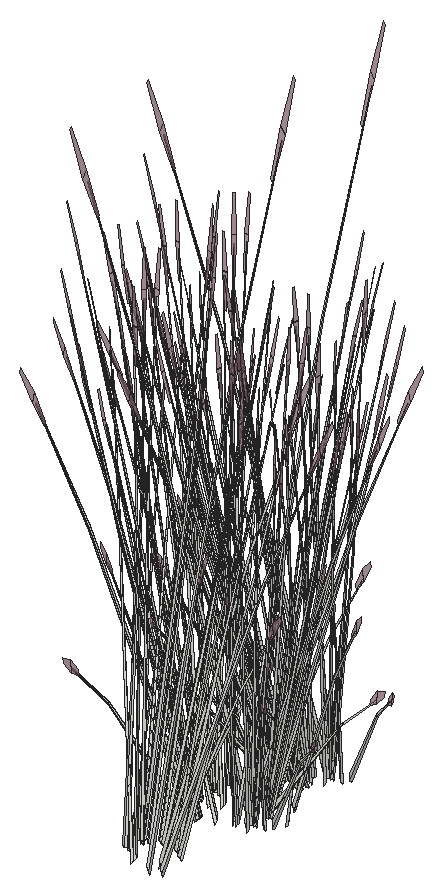
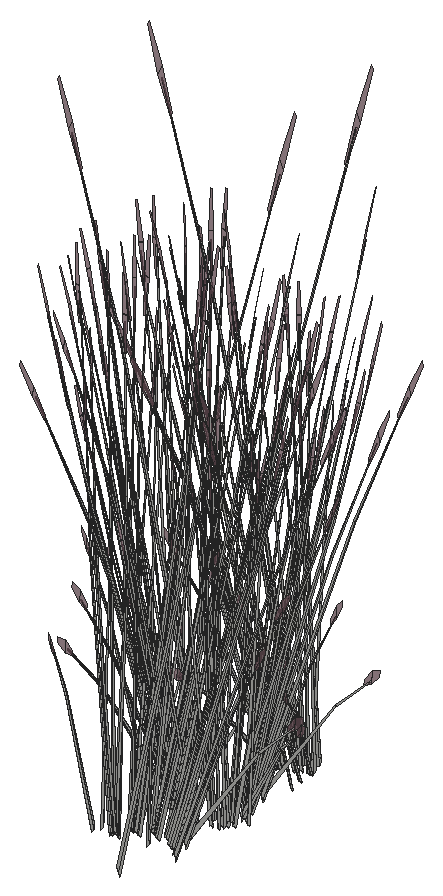
# SketchUp Ruby script. Lengths in inches.
U = 1.inch
M = Sketchup.active_model
def pt(a) = Geom::Point3d.new(a.map { |v| v * U })
def face(e, loops, mat)
  f = e.add_face(loops[0].map { |a| pt(a) })
  loops[1..].each { |l| e.add_face(l.map { |a| pt(a) }).erase! }
  f.material = f.back_material = mat if mat
  f
end
# faces: each face lists its corners as indices into pts; further lists are holes
def faces(e, pts, list, mat = nil) = list.each { |f| face(e, (f[0].is_a?(Array) ? f : [f]).map { |l| l.map { |i| pts[i] } }, mat) }
# xy, xz, yz: faces in a plane at the given z, y or x. An outline is a flat list of corners, or four numbers for a rectangle; further outlines are holes
def ring(l) = l.size == 4 ? [[l[0], l[1]], [l[2], l[1]], [l[2], l[3]], [l[0], l[3]]] : l.each_slice(2).to_a
def flat(e, list, mat, &to3) = list.each { |f| face(e, (f[0].is_a?(Array) ? f : [f]).map { |l| ring(l).map { |u, v| to3.(u, v) } }, mat) }
def xy(e, z, list, mat = nil) = flat(e, list, mat) { |x, y| [x, y, z] }
def xz(e, y, list, mat = nil) = flat(e, list, mat) { |x, z| [x, y, z] }
def yz(e, x, list, mat = nil) = flat(e, list, mat) { |y, z| [x, y, z] }
def lines(e, pts, list) = list.each { |a, b| e.add_line(pt(pts[a]), pt(pts[b])) }
# prism: a flat outline (further loops are holes) pulled along v
def prism(e, loops, v, mat = nil)
  f = face(e, loops, mat); d = Geom::Vector3d.new(v.map { |x| x * U })
  f.pushpull(f.normal.samedirection?(d) ? d.length : -d.length)
end
def box(e, o, s, mat = nil) = prism(e, [[o, [o[0] + s[0], o[1], o[2]], [o[0] + s[0], o[1] + s[1], o[2]], [o[0], o[1] + s[1], o[2]]]], [0, 0, s[2]], mat)
def at(x, y, z, deg = 0) = Geom::Transformation.translation(pt([x, y, z])) * Geom::Transformation.rotation(ORIGIN, Z_AXIS, deg.degrees)
def axes(o, x, y, z) = Geom::Transformation.new([*x, 0, *y, 0, *z, 0, *pt(o).to_a, 1])
def part(name) = M.definitions.add(name)
# library, detail: a bought-in or finely detailed component or shape, given as its bounding box
def library(name, o, s) = part(name).tap { |d| box(d.entities, o, s) }
def detail(e, o, s) = box(e.add_group.entities, o, s)
def put(e, d, t, mat = nil) = e.add_instance(d, t).tap { |i| i.material = mat if mat }
def group(e, t, mat = nil) = e.add_group.tap { |g| g.transformation = t; g.material = mat if mat }.entities
root = M.entities
M.materials.add("LightPink_Translucent").color = [144, 107, 117]
M.materials["LightPink_Translucent"].alpha = 0.75
c1 = part("blade")
p = [[2.15,0.21,22],[0,0.17,0],[0.09,0.45,0],[2.18,0.31,22],[2.29,0.31,22],[0.38,0.45,0],
  [2.48,0.24,33],[2.49,0.24,33],[2.48,0.22,33]]
faces(c1.entities,p,[[0,1,2,3],[4,5,2,3],[6,3,4,7],[8,0,3,6]])
c2 = part("seeds")
p = [[0.3,-0.1,1.38],[-0.01,-0.03,1.59],[-0.01,-0.03,0.03],[0.14,-0.07,-0.07],[0.29,-0.03,3],[0.15,0.01,3.11]]
faces(c2.entities,p,[[0,1,2,3],[1,0,4,5]],"LightPink_Translucent")
c3 = part("blade with seeds")
put(c3.entities,c1,at(0,0,0))
put(c3.entities,c2,axes([2.4,0.25,30.99],[1.5799,-0.05474,1.17369],[-0.12525,1.92788,0.29478],[-0.07173,-0.02425,1.56792]))
put(root,c3,axes([428.51,484.51,154],[0.18625,-0.29962,0.05432],[0.26523,0.17444,0.42765],[-0.08575,-0.09606,0.65209]))
put(root,c3,axes([427.57,485.1,153.27],[0.15222,0.08126,1.44779],[-0.31502,0.34091,0.11706],[-0.19634,-0.15379,0.61892]))
put(root,c3,axes([429.86,479.9,153.27],[-0.15222,-0.08126,1.44779],[0.31502,-0.34091,0.11706],[0.19634,0.15379,0.61892]))
put(root,c3,axes([429.88,478.83,153.78],[-0.35411,-0.24507,1.16821],[0.37391,-0.38156,0.50405],[0.11425,0.22994,1.12919]))
put(root,c3,axes([427.33,479.87,154.25],[0.37908,0.26007,-0.10273],[-0.21839,0.37663,-0.57019],[-0.1071,0.13092,0.8664]))
put(root,c3,axes([428.31,484.86,153.95],[-0.40438,0.11212,-0.43168],[-0.07074,-0.4246,-0.33437],[-0.10862,-0.12168,0.82598]))
put(root,c3,axes([430.35,484.95,154],[0.29182,0.32181,0.40553],[-0.3099,0.27755,0.33437],[0.05383,-0.15098,0.83914]))
put(root,c3,axes([429.61,481.22,154.25],[0.2442,-0.40372,-0.10273],[0.35364,0.23259,-0.57019],[0.12293,0.11406,0.8664]))
put(root,c3,axes([428.59,484.48,154.59],[-0.2735,0.45217,-0.11506],[-0.39608,-0.2605,-0.63862],[-0.13768,-0.12775,0.97037]))
put(root,c3,axes([430.46,484.98,154],[0.33677,0.02198,0.05432],[-0.00923,0.33185,0.42765],[0.03524,-0.12712,0.65209]))
put(root,c3,axes([427.84,479.75,153.27],[0.10236,-0.14492,1.44779],[0.25844,0.39118,0.11706],[-0.17726,0.17814,0.61892]))
put(root,c3,axes([427.52,480.18,153.95],[0.10528,0.43067,-0.43168],[-0.39868,0.07534,-0.33437],[-0.11425,0.11568,0.82598]))
put(root,c3,axes([430.7,485.87,154.21],[0.21406,-0.37215,-0.60019],[0.37511,0.26448,0.07243],[0.12781,-0.13483,0.84903]))
put(root,c3,axes([430.6875,485.7,153.95],[-0.10528,-0.43067,-0.43168],[0.39868,-0.07534,-0.33437],[0.11425,-0.11568,0.82598]))
put(root,c3,axes([429.29,481.55,153.98],[0.00121,-0.0571,1.49853],[0.35119,-0.25193,-0.1416],[0.12199,0.08992,0.26519]))
put(root,c3,axes([427.75,480.9,154],[-0.33677,-0.02198,0.05432],[0.00923,-0.33185,0.42765],[-0.03524,0.12712,0.65209]))
put(root,c3,axes([427.85,480.93,154],[-0.29182,-0.32181,0.40553],[0.3099,-0.27755,0.33437],[-0.05383,0.15098,0.83914]))
put(root,c3,axes([429.9,481.02,153.95],[0.40438,-0.11212,-0.43168],[0.07074,0.4246,-0.33437],[0.10862,0.12168,0.82598]))
put(root,c3,axes([427.54,484.35,153.98],[-0.08817,-0.00333,1.47793],[-0.28072,0.33293,-0.23373],[-0.14978,-0.06803,0.11853]))
put(root,c3,axes([430.875,486.01,154.25],[-0.37908,-0.26007,-0.10273],[0.21839,-0.37663,-0.57019],[0.1071,-0.13092,0.8664]))
put(root,c3,axes([429.31,487.43,152.81],[0.35414,0.19019,1.27785],[-0.34693,0.40974,0.50532],[-0.1554,-0.24285,1.07126]))
put(root,c3,axes([429.7,481.36,154],[-0.18625,0.29962,0.05432],[-0.26523,-0.17444,0.42765],[0.08575,0.09606,0.65209]))
put(root,c3,axes([431.81,485.89,153.98],[-0.05353,-0.00358,1.49853],[-0.22227,-0.38383,-0.1416],[0.08926,-0.1262,0.26519]))
put(root,c3,axes([429.78,481.28,154],[-0.4076,0.10824,0.40553],[-0.07074,-0.4246,0.33437],[0.09586,0.12514,0.83914]))
put(root,c3,axes([427.77,480.11,153.27],[0.0763,-0.16212,1.44779],[0.3201,0.3355,0.11706],[-0.1444,0.2091,0.61892]))
put(root,c3,axes([430.98,485.74,153.82],[0.35672,-0.06741,-0.29918],[0.09419,0.38534,0.38624],[0.10222,-0.1035,0.73904]))
put(root,c3,axes([427.63,485.1,154],[0.02064,-0.35866,0.05432],[0.3116,0.00983,0.42765],[-0.11936,-0.03753,0.65209]))
put(root,c3,axes([428.66,481.41,154],[-0.30197,0.1603,0.05432],[-0.1478,-0.29231,0.42765],[0.02916,0.12885,0.65209]))
put(root,c3,axes([427.85,481.02,153.82],[-0.27728,0.24833,-0.29918],[-0.26248,-0.28355,0.38624],[-0.03994,0.14407,0.73904]))
put(root,c3,axes([426.9,480.95,153.98],[-0.01019,0.09334,1.47793],[0.28908,0.3247,-0.23373],[-0.07568,0.15355,0.11853]))
put(root,c3,axes([427.82,480.74,154.56],[0.45039,0.02337,-0.11403],[-0.01231,0.44247,-0.63292],[-0.03129,0.17041,0.9617]))
put(root,c3,axes([427.51,485.21,153.82],[-0.23317,-0.29531,-0.29918],[0.26625,-0.27955,0.38624],[-0.13527,-0.04253,0.73904]))
put(root,c3,axes([428.66,481.23,154.25],[0.40102,-0.2196,-0.10273],[0.19707,0.38974,-0.57019],[0.05291,0.16424,0.8664]))
put(root,c3,axes([428.13,480.91,154.23],[0.29336,0.31691,-0.47917],[-0.3099,0.27755,-0.37115],[-0.04464,0.16102,0.91684]))
put(root,c3,axes([427.76,485.41,154.21],[-0.40965,-0.01136,-0.60019],[0.02751,-0.47821,0.07243],[-0.17355,-0.05047,0.84903]))
put(root,c3,axes([429,481.21,153.95],[0.40284,0.11824,-0.43168],[-0.13808,0.40538,-0.33437],[0.03694,0.16321,0.82598]))
put(root,c3,axes([429.23,480.375,153.27],[-0.09368,-0.15143,1.44779],[0.43286,-0.12749,0.11706],[0.09783,0.23774,0.61892]))
put(root,c3,axes([431.01,485.91,154],[0.28133,0.19836,0.05432],[-0.16379,0.28248,0.42765],[0.0902,-0.09132,0.65209]))
put(root,c3,axes([428.82,481.46,153.82],[-0.12355,0.36271,-0.29918],[-0.36044,-0.10579,0.38624],[0.03305,0.14603,0.73904]))
put(root,c3,axes([430.93,485.83,154],[0.10163,0.43409,0.40553],[-0.39868,0.07534,0.33437],[0.1175,-0.10209,0.83914]))
put(root,c3,axes([432.01,486.35,153.98],[0.05687,-0.07184,1.47793],[-0.07279,-0.44069,-0.23373],[0.14268,-0.08356,0.11853]))
put(root,c3,axes([428.04,480.76,154.51],[-0.01066,0.43628,-0.66621],[-0.44902,-0.0293,0.0804],[-0.04739,0.18483,0.94242]))
put(root,c3,axes([426.87,481.91,153.98],[0.04649,-0.02848,1.49853],[0.38427,0.18941,-0.1416],[-0.00903,0.15771,0.26519]))
put(root,c3,axes([427.2,484.63,153.98],[0.03038,0.04707,1.49853],[-0.14646,0.42312,-0.1416],[-0.14833,0.00306,0.26519]))
put(root,c3,axes([428.46,480.45,153.27],[-0.01003,-0.18103,1.44779],[0.43473,0.12009,0.11706],[-0.02689,0.25798,0.61892]))
put(root,c3,axes([427.625,485.51,153.95],[-0.29757,0.31243,-0.43168],[-0.2606,-0.33005,-0.33437],[-0.15119,-0.04754,0.82598]))
put(root,c3,axes([428.5625,482.1,153.98],[0.05195,0.07595,1.47793],[0.41921,0.02984,-0.23373],[0.04216,0.1675,0.11853]))
put(root,c3,axes([427.78,485.18,154.25],[-0.02194,0.47967,-0.10273],[-0.41546,-0.01311,-0.57019],[-0.16001,-0.03332,0.8664]))
put(root,c3,axes([430.89,487.02,154.25],[-0.20619,-0.42709,-0.10273],[0.36595,-0.20988,-0.57019],[0.15422,-0.05635,0.8664]))
put(root,c3,axes([430.87,486.65,153.95],[0.11102,-0.42903,-0.43168],[0.38064,0.14706,-0.33437],[0.15325,-0.03934,0.82598]))
put(root,c3,axes([427.25,485.84,153.27],[0.16998,-0.01068,1.44779],[-0.11276,0.46299,0.11706],[-0.24224,-0.02864,0.61892]))
put(root,c3,axes([430.8,486.81,154.21],[0.3601,-0.20831,-0.60019],[0.20068,0.4288,0.07243],[0.17399,-0.04871,0.84903]))
put(root,c3,axes([427.89,481.375,152.84],[0.009,-0.24349,1.30391],[0.40497,0.12861,0.18019],[-0.03509,0.2595,0.61571]))
put(root,c3,axes([427.18,486.19,154],[0.11578,-0.43006,0.40553],[0.38064,0.14706,0.33437],[-0.14969,0.02584,0.83914]))
put(root,c3,axes([427.15,486.08,154],[-0.15051,-0.3216,0.05432],[0.27447,-0.15741,0.42765],[-0.12099,0.03106,0.65209]))
put(root,c3,axes([431.1,486.85,153.82],[0.34057,0.13158,-0.29918],[-0.09933,0.38387,0.38624],[0.13712,-0.0352,0.73904]))
put(root,c3,axes([427.1,486.24,153.82],[-0.34057,-0.13158,-0.29918],[0.09933,-0.38387,0.38624],[-0.13712,0.0352,0.73904]))
put(root,c3,axes([428.2,490.79,153.27],[0.09368,0.15143,1.44779],[-0.43286,0.12749,0.11706],[-0.09783,-0.23774,0.61892]))
put(root,c3,axes([430.18,486.375,153.27],[-0.16998,0.01068,1.44779],[0.11276,-0.46299,0.11706],[0.24224,0.02864,0.61892]))
put(root,c3,axes([428.91,489.79,153.98],[-0.06268,-0.06613,1.47793],[-0.4183,0.04193,-0.23373],[-0.06676,-0.15817,0.11853]))
put(root,c3,axes([431.05,487.01,154],[0.15051,0.3216,0.05432],[-0.27447,0.15741,0.42765],[0.12099,-0.03106,0.65209]))
put(root,c3,axes([429.35,490.9,154.21],[-0.19559,-0.38351,-0.60019],[0.40262,-0.21373,0.07243],[-0.04574,-0.1853,0.84903]))
put(root,c3,axes([431.03,486.9,154],[-0.11578,0.43006,0.40553],[-0.38064,-0.14706,0.33437],[0.14969,-0.02584,0.83914]))
put(root,c3,axes([430.17,491.28,154.21],[0.01066,-0.43628,-0.60019],[0.44902,0.0293,0.07243],[0.04739,-0.18483,0.84903]))
put(root,c3,axes([428.14,486.17,152.82],[0.11649,-0.06823,1.49584],[0.04017,0.47639,0.11706],[-0.25231,0.06321,0.53462]))
put(root,c3,axes([430.79,490.6,153.98],[-0.00396,-0.09387,1.47793],[-0.33411,-0.2713,-0.23373],[0.05166,-0.16446,0.11853]))
put(root,c3,axes([429.39,490.58,153.82],[0.12355,-0.36271,-0.29918],[0.36044,0.10579,0.38624],[-0.03305,-0.14603,0.73904]))
put(root,c3,axes([429.66,491.06,153.27],[-0.0763,0.16212,1.44779],[-0.3201,-0.3355,0.11706],[0.1444,-0.2091,0.61892]))
put(root,c3,axes([430.7,490.26,153.98],[-0.04162,0.03603,1.49853],[-0.40776,-0.12155,-0.1416],[-0.01476,-0.15722,0.26519]))
put(root,c3,axes([429.21,490.83,153.95],[-0.40284,-0.11824,-0.43168],[0.13808,-0.40538,-0.33437],[-0.03694,-0.16321,0.82598]))
put(root,c3,axes([431.71,488.29,153.98],[-0.03706,-0.04129,1.49853],[0.08106,-0.44261,-0.1416],[0.14596,-0.02828,0.26519]))
put(root,c3,axes([430.08,491.13,153.95],[-0.29336,-0.31691,-0.43168],[0.3099,-0.27755,-0.33437],[0.04464,-0.16102,0.82598]))
put(root,c3,axes([426.89,486.49,153.98],[-0.06692,0.06124,1.47793],[0.00569,0.44742,-0.23373],[-0.15339,0.05818,0.11853]))
put(root,c3,axes([427.34,486.43,153.95],[-0.11102,0.42903,-0.43168],[-0.38064,-0.14706,-0.33437],[-0.15325,0.03934,0.82598]))
put(root,c3,axes([427.32,486.07,154.25],[0.20619,0.42709,-0.10273],[-0.36595,0.20988,-0.57019],[-0.15422,0.05635,0.8664]))
put(root,c3,axes([431.39,487.92,153.32],[-0.07843,-0.39649,-0.0295],[0.37072,-0.09115,-0.13375],[0.07742,0.02514,0.44114]))
put(root,c3,axes([428.49,489.57,153.98],[-0.00765,0.05653,1.49853],[-0.37706,0.20517,-0.1416],[-0.11096,-0.10488,0.26519]))
put(root,c3,axes([430.43,487.91,154.25],[0.02194,-0.47967,-0.10273],[0.41546,0.01311,-0.57019],[0.16001,0.03332,0.8664]))
put(root,c3,axes([429.43,490.66,154],[0.4038,0.12331,0.40553],[-0.13808,0.40538,0.33437],[-0.02427,-0.15942,0.83914]))
put(root,c3,axes([429.55,490.81,154.25],[-0.40102,0.2196,-0.10273],[-0.19707,-0.38974,-0.57019],[-0.05291,-0.16424,0.8664]))
put(root,c3,axes([430.38,491.3,154.25],[-0.45039,-0.02337,-0.10273],[0.01231,-0.44247,-0.57019],[0.03129,-0.17041,0.8664]))
put(root,c3,axes([430.35,491.02,153.82],[0.27728,-0.24833,-0.29918],[0.26248,0.28355,0.38624],[0.03994,-0.14407,0.73904]))
put(root,c3,axes([429.54,490.63,154],[0.30197,-0.1603,0.05432],[0.1478,0.29231,0.42765],[-0.02916,-0.12885,0.65209]))
put(root,c3,axes([428.47,491.01,154.21],[-0.34944,-0.22798,-0.60019],[0.24834,-0.39949,0.07243],[-0.1266,-0.13612,0.84903]))
put(root,c3,axes([428.35,490.71,153.82],[-0.06329,-0.37991,-0.29918],[0.36182,-0.10032,0.38624],[-0.09718,-0.10887,0.73904]))
put(root,c3,axes([430.79,487.62,153.98],[0.08791,-0.00798,1.47793],[0.24113,-0.36643,-0.23373],[0.15637,0.04837,0.11853]))
put(root,c3,axes([427.27,487.26,154],[-0.10163,-0.43409,0.40553],[0.39868,-0.07534,0.33437],[-0.1175,0.10209,0.83914]))
put(root,c3,axes([427.19,487.18,154],[-0.28133,-0.19836,0.05432],[0.16379,-0.28248,0.42765],[-0.0902,0.09132,0.65209]))
put(root,c3,axes([427.32,486.66,153.27],[0.14219,-0.09977,1.44779],[0.11971,0.461,0.11706],[-0.22323,0.10419,0.61892]))
put(root,c3,axes([428.51,490.68,154],[0.18625,-0.29962,0.05432],[0.26523,0.17444,0.42765],[-0.08575,-0.09606,0.65209]))
put(root,c3,axes([427.57,491.26,153.27],[0.15222,0.08126,1.44779],[-0.31502,0.34091,0.11706],[-0.19634,-0.15379,0.61892]))
put(root,c3,axes([430.45,487.68,154.21],[0.40965,0.01136,-0.60019],[-0.02751,0.47821,0.07243],[0.17355,0.05047,0.84903]))
put(root,c3,axes([428.31,491.02,153.95],[-0.40438,0.11212,-0.43168],[-0.07074,-0.4246,-0.33437],[-0.10862,-0.12168,0.82598]))
put(root,c3,axes([430.35,491.11,154],[0.29182,0.32181,0.40553],[-0.3099,0.27755,0.33437],[0.05383,-0.15098,0.83914]))
put(root,c3,axes([428.59,490.65,154.59],[-0.2735,0.45217,-0.11506],[-0.39608,-0.2605,-0.63862],[-0.13768,-0.12775,0.97037]))
put(root,c3,axes([430.46,491.14,154],[0.33677,0.02198,0.05432],[-0.00923,0.33185,0.42765],[0.03524,-0.12712,0.65209]))
put(root,c3,axes([426.14,486.95,153.98],[0.0523,0.01265,1.49853],[0.16179,0.41674,-0.1416],[-0.10706,0.10938,0.26519]))
put(root,c3,axes([430.7,492.04,154.21],[0.21406,-0.37215,-0.60019],[0.37511,0.26448,0.07243],[0.12781,-0.13483,0.84903]))
put(root,c3,axes([430.69,487.875,153.82],[0.23317,0.29531,-0.29918],[-0.26625,0.27955,0.38624],[0.13527,0.04253,0.73904]))
put(root,c3,axes([430.6875,491.86,153.95],[-0.10528,-0.43067,-0.43168],[0.39868,-0.07534,-0.33437],[0.11425,-0.11568,0.82598]))
put(root,c3,axes([430.57,487.99,154],[-0.02064,0.35866,0.05432],[-0.3116,-0.00983,0.42765],[0.11936,0.03753,0.65209]))
put(root,c3,axes([427.23,487.35,153.82],[-0.35672,0.06741,-0.29918],[-0.09419,-0.38534,0.38624],[-0.10222,0.1035,0.73904]))
put(root,c3,axes([430.6,487.875,154],[-0.30217,0.31079,0.40553],[-0.2606,-0.33005,0.33437],[0.14177,0.05733,0.83914]))
put(root,c3,axes([427.54,490.51,153.98],[-0.08817,-0.00333,1.47793],[-0.28072,0.33293,-0.23373],[-0.14978,-0.06803,0.11853]))
put(root,c3,axes([430.875,492.17,154.25],[-0.37908,-0.26007,-0.10273],[0.21839,-0.37663,-0.57019],[0.1071,-0.13092,0.8664]))
put(root,c3,axes([429.31,493.59,152.81],[0.35414,0.19019,1.27785],[-0.34693,0.40974,0.50532],[-0.1554,-0.24285,1.07126]))
put(root,c3,axes([431.81,492.06,153.98],[-0.05353,-0.00358,1.49853],[-0.22227,-0.38383,-0.1416],[0.08926,-0.1262,0.26519]))
put(root,c3,axes([429.86,487.12,153.27],[-0.15222,-0.08126,1.44779],[0.31502,-0.34091,0.11706],[0.19634,0.15379,0.61892]))
put(root,c3,axes([429.88,486.05,153.78],[-0.35411,-0.24507,1.16821],[0.37391,-0.38156,0.50405],[0.11425,0.22994,1.12919]))
put(root,c3,axes([427.33,487.08,154.25],[0.37908,0.26007,-0.10273],[-0.21839,0.37663,-0.57019],[-0.1071,0.13092,0.8664]))
put(root,c3,axes([429.61,488.43,154.25],[0.2442,-0.40372,-0.10273],[0.35364,0.23259,-0.57019],[0.12293,0.11406,0.8664]))
put(root,c3,axes([430.98,491.91,153.82],[0.35672,-0.06741,-0.29918],[0.09419,0.38534,0.38624],[0.10222,-0.1035,0.73904]))
put(root,c3,axes([427.84,486.97,153.27],[0.10236,-0.14492,1.44779],[0.25844,0.39118,0.11706],[-0.17726,0.17814,0.61892]))
put(root,c3,axes([427.63,491.27,154],[0.02064,-0.35866,0.05432],[0.3116,0.00983,0.42765],[-0.11936,-0.03753,0.65209]))
put(root,c3,axes([427.52,487.39,153.95],[0.10528,0.43067,-0.43168],[-0.39868,0.07534,-0.33437],[-0.11425,0.11568,0.82598]))
put(root,c3,axes([427.51,491.38,153.82],[-0.23317,-0.29531,-0.29918],[0.26625,-0.27955,0.38624],[-0.13527,-0.04253,0.73904]))
put(root,c3,axes([429.29,488.77,153.98],[0.00121,-0.0571,1.49853],[0.35119,-0.25193,-0.1416],[0.12199,0.08992,0.26519]))
put(root,c3,axes([427.75,488.11,154],[-0.33677,-0.02198,0.05432],[0.00923,-0.33185,0.42765],[-0.03524,0.12712,0.65209]))
put(root,c3,axes([427.85,488.14,154],[-0.29182,-0.32181,0.40553],[0.3099,-0.27755,0.33437],[-0.05383,0.15098,0.83914]))
put(root,c3,axes([429.9,488.23,153.95],[0.40438,-0.11212,-0.43168],[0.07074,0.4246,-0.33437],[0.10862,0.12168,0.82598]))
put(root,c3,axes([427.76,491.58,154.21],[-0.40965,-0.01136,-0.60019],[0.02751,-0.47821,0.07243],[-0.17355,-0.05047,0.84903]))
put(root,c3,axes([429.7,488.58,154],[-0.18625,0.29962,0.05432],[-0.26523,-0.17444,0.42765],[0.08575,0.09606,0.65209]))
put(root,c3,axes([431.01,492.08,154],[0.28133,0.19836,0.05432],[-0.16379,0.28248,0.42765],[0.0902,-0.09132,0.65209]))
put(root,c3,axes([430.93,491.99,154],[0.10163,0.43409,0.40553],[-0.39868,0.07534,0.33437],[0.1175,-0.10209,0.83914]))
put(root,c3,axes([432.01,492.52,153.98],[0.05687,-0.07184,1.47793],[-0.07279,-0.44069,-0.23373],[0.14268,-0.08356,0.11853]))
put(root,c3,axes([429.78,488.49,154],[-0.4076,0.10824,0.40553],[-0.07074,-0.4246,0.33437],[0.09586,0.12514,0.83914]))
put(root,c3,axes([427.77,487.32,153.27],[0.0763,-0.16212,1.44779],[0.3201,0.3355,0.11706],[-0.1444,0.2091,0.61892]))
put(root,c3,axes([427.2,490.8,153.98],[0.03038,0.04707,1.49853],[-0.14646,0.42312,-0.1416],[-0.14833,0.00306,0.26519]))
put(root,c3,axes([428.66,488.62,154],[-0.30197,0.1603,0.05432],[-0.1478,-0.29231,0.42765],[0.02916,0.12885,0.65209]))
put(root,c3,axes([427.85,488.24,153.82],[-0.27728,0.24833,-0.29918],[-0.26248,-0.28355,0.38624],[-0.03994,0.14407,0.73904]))
